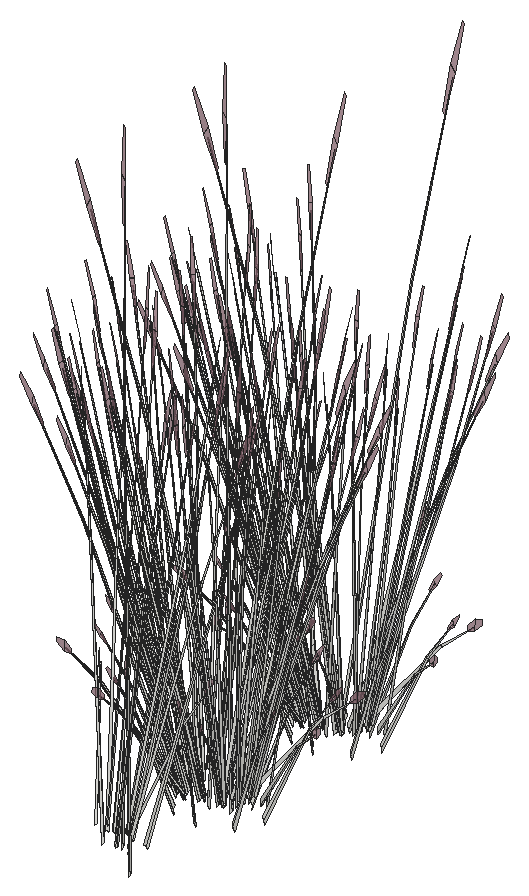
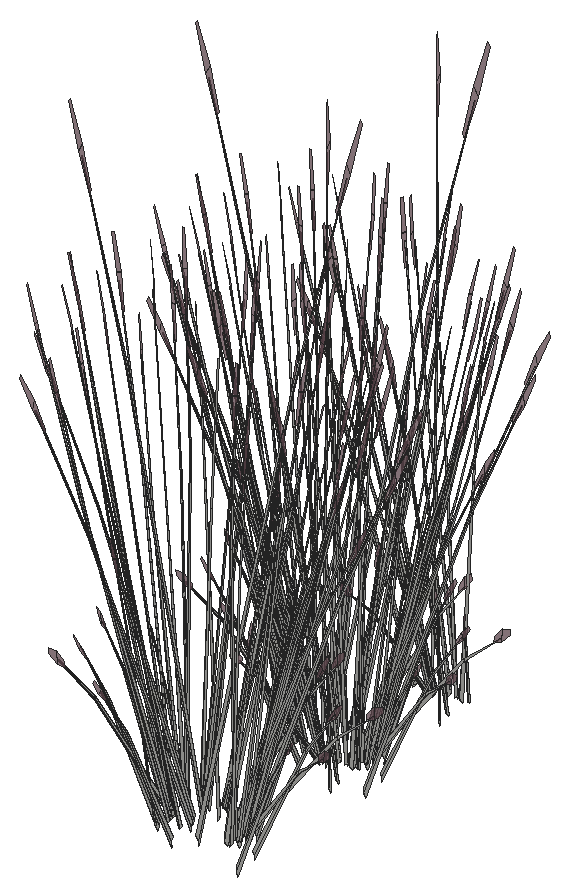
# SketchUp Ruby script. Lengths in inches.
U = 1.inch
M = Sketchup.active_model
def pt(a) = Geom::Point3d.new(a.map { |v| v * U })
def face(e, loops, mat)
  f = e.add_face(loops[0].map { |a| pt(a) })
  loops[1..].each { |l| e.add_face(l.map { |a| pt(a) }).erase! }
  f.material = f.back_material = mat if mat
  f
end
# faces: each face lists its corners as indices into pts; further lists are holes
def faces(e, pts, list, mat = nil) = list.each { |f| face(e, (f[0].is_a?(Array) ? f : [f]).map { |l| l.map { |i| pts[i] } }, mat) }
# xy, xz, yz: faces in a plane at the given z, y or x. An outline is a flat list of corners, or four numbers for a rectangle; further outlines are holes
def ring(l) = l.size == 4 ? [[l[0], l[1]], [l[2], l[1]], [l[2], l[3]], [l[0], l[3]]] : l.each_slice(2).to_a
def flat(e, list, mat, &to3) = list.each { |f| face(e, (f[0].is_a?(Array) ? f : [f]).map { |l| ring(l).map { |u, v| to3.(u, v) } }, mat) }
def xy(e, z, list, mat = nil) = flat(e, list, mat) { |x, y| [x, y, z] }
def xz(e, y, list, mat = nil) = flat(e, list, mat) { |x, z| [x, y, z] }
def yz(e, x, list, mat = nil) = flat(e, list, mat) { |y, z| [x, y, z] }
def lines(e, pts, list) = list.each { |a, b| e.add_line(pt(pts[a]), pt(pts[b])) }
# prism: a flat outline (further loops are holes) pulled along v
def prism(e, loops, v, mat = nil)
  f = face(e, loops, mat); d = Geom::Vector3d.new(v.map { |x| x * U })
  f.pushpull(f.normal.samedirection?(d) ? d.length : -d.length)
end
def box(e, o, s, mat = nil) = prism(e, [[o, [o[0] + s[0], o[1], o[2]], [o[0] + s[0], o[1] + s[1], o[2]], [o[0], o[1] + s[1], o[2]]]], [0, 0, s[2]], mat)
def at(x, y, z, deg = 0) = Geom::Transformation.translation(pt([x, y, z])) * Geom::Transformation.rotation(ORIGIN, Z_AXIS, deg.degrees)
def axes(o, x, y, z) = Geom::Transformation.new([*x, 0, *y, 0, *z, 0, *pt(o).to_a, 1])
def part(name) = M.definitions.add(name)
# library, detail: a bought-in or finely detailed component or shape, given as its bounding box
def library(name, o, s) = part(name).tap { |d| box(d.entities, o, s) }
def detail(e, o, s) = box(e.add_group.entities, o, s)
def put(e, d, t, mat = nil) = e.add_instance(d, t).tap { |i| i.material = mat if mat }
def group(e, t, mat = nil) = e.add_group.tap { |g| g.transformation = t; g.material = mat if mat }.entities
root = M.entities
M.materials.add("LightPink_Translucent").color = [144, 107, 117]
M.materials["LightPink_Translucent"].alpha = 0.75
c1 = part("blade")
p = [[2.15,0.21,22],[0,0.17,0],[0.09,0.45,0],[2.18,0.31,22],[2.29,0.31,22],[0.38,0.45,0],
  [2.48,0.24,33],[2.49,0.24,33],[2.48,0.22,33]]
faces(c1.entities,p,[[0,1,2,3],[4,5,2,3],[6,3,4,7],[8,0,3,6]])
c2 = part("seeds")
p = [[0.3,-0.1,1.38],[-0.01,-0.03,1.59],[-0.01,-0.03,0.03],[0.14,-0.07,-0.07],[0.29,-0.03,3],[0.15,0.01,3.11]]
faces(c2.entities,p,[[0,1,2,3],[1,0,4,5]],"LightPink_Translucent")
c3 = part("blade with seeds")
put(c3.entities,c1,at(0,0,0))
put(c3.entities,c2,axes([2.4,0.25,30.99],[1.5799,-0.05474,1.17369],[-0.12525,1.92788,0.29478],[-0.07173,-0.02425,1.56792]))
put(root,c3,axes([334.74,295.48,50.51],[-0.01379,-0.36791,1.24828],[0.62424,0.09537,0.52853],[-0.14764,0.20132,1.17828]))
put(root,c3,axes([334.79,296.9,52.14],[0.49824,-0.09289,-0.45151],[0.08716,0.35177,-0.34973],[0.13382,0.10081,0.86392]))
put(root,c3,axes([332.16,296.15,51.43],[0.09401,-0.13431,1.51428],[0.3944,0.27795,0.12244],[-0.17792,0.17323,0.64734]))
put(root,c3,axes([332.27,296.91,52],[-0.34164,0.20573,-0.31292],[-0.3234,-0.23491,0.40398],[-0.04921,0.11936,0.77298]))
put(root,c3,axes([331.09,296.85,52.17],[-0.01255,0.07733,1.54581],[0.35618,0.269,-0.24447],[-0.09325,0.12721,0.12397]))
put(root,c3,axes([333.25,297.08,52.45],[0.49409,-0.18193,-0.10745],[0.24281,0.32289,-0.59638],[0.06519,0.13607,0.90619]))
put(root,c3,axes([332.48,297.71,50.44],[-0.01307,-0.23234,1.01491],[0.32652,0.16572,0.74569],[-0.06422,0.11074,0.22354]))
put(root,c3,axes([332.61,296.8125,52.42],[0.36145,0.26255,-0.50118],[-0.38183,0.22994,-0.3882],[-0.055,0.1334,0.95895]))
put(root,c3,axes([333.68,297.07,52.14],[0.49634,0.09796,-0.45151],[-0.17013,0.33585,-0.34973],[0.04551,0.13522,0.86392]))
put(root,c3,axes([333.96,296.37,51.43],[-0.11542,-0.12546,1.51428],[0.53333,-0.10562,0.12244],[0.12054,0.19696,0.64734]))
put(root,c3,axes([333.45,297.27,52],[-0.15222,0.30049,-0.31292],[-0.44409,-0.08764,0.40398],[0.04072,0.12098,0.77298]))
put(root,c3,axes([332.49,296.69,52.72],[-0.01314,0.36145,-0.69681],[-0.55324,-0.02428,0.08409],[-0.05838,0.15313,0.9857]))
put(root,c3,axes([332.69,303.4,51.43],[0.11542,0.12546,1.51428],[-0.53333,0.10562,0.12244],[-0.12054,-0.19696,0.64734]))
put(root,c3,axes([333.02,296.43,51.43],[-0.01236,-0.14998,1.51428],[0.53562,0.09949,0.12244],[-0.03313,0.21373,0.64734]))
put(root,c3,axes([333.57,302.57,52.17],[-0.07723,-0.05479,1.54581],[-0.51538,0.03473,-0.24447],[-0.08225,-0.13104,0.12397]))
put(root,c3,axes([334.11,303.49,52.4],[-0.24099,-0.31773,-0.62776],[0.49607,-0.17707,0.07576],[-0.05635,-0.15352,0.88802]))
put(root,c3,axes([333.5,297,52.4],[0.24099,0.31773,-0.62776],[-0.49607,0.17707,0.07576],[0.05635,0.15352,0.88802]))
put(root,c3,axes([333.14,297.8,52.17],[0.064,0.06292,1.54581],[0.51651,0.02472,-0.24447],[0.05194,0.13877,0.12397]))
put(root,c3,axes([335.12,303.8,52.4],[0.01314,-0.36145,-0.62776],[0.55324,0.02428,0.07576],[0.05838,-0.15313,0.88802]))
put(root,c3,axes([335.89,303.24,52.17],[-0.00487,-0.07777,1.54581],[-0.41166,-0.22476,-0.24447],[0.06364,-0.13625,0.12397]))
put(root,c3,axes([334.16,303.22,52],[0.15222,-0.30049,-0.31292],[0.44409,0.08764,0.40398],[-0.04072,-0.12098,0.77298]))
put(root,c3,axes([334.5,303.62,51.43],[-0.09401,0.13431,1.51428],[-0.3944,-0.27795,0.12244],[0.17792,-0.17323,0.64734]))
put(root,c3,axes([333.93,303.43,52.14],[-0.49634,-0.09796,-0.45151],[0.17013,-0.33585,-0.34973],[-0.04551,-0.13522,0.86392]))
put(root,c3,axes([334.24,302.59,50.44],[0.06477,0.22786,1.01491],[-0.35932,-0.1262,0.74569],[0.03867,-0.11667,0.22354]))
put(root,c3,axes([332.31,297.2,50.97],[0.01109,-0.20172,1.3638],[0.49896,0.10655,0.18846],[-0.04323,0.21498,0.64398]))
put(root,c3,axes([335.01,303.68,52.14],[-0.36145,-0.26255,-0.45151],[0.38183,-0.22994,-0.34973],[0.055,-0.1334,0.86392]))
put(root,c3,axes([334.36,303.41,52.45],[-0.49409,0.18193,-0.10745],[-0.24281,-0.32289,-0.59638],[-0.06519,-0.13607,0.90619]))
put(root,c3,axes([335.38,303.82,52.45],[-0.55492,-0.01936,-0.10745],[0.01517,-0.36657,-0.59638],[0.03855,-0.14118,0.90619]))
put(root,c3,axes([335.35,303.59,52],[0.34164,-0.20573,-0.31292],[0.3234,0.23491,0.40398],[0.04921,-0.11936,0.77298]))
put(root,c3,axes([332.39,302.86,50.44],[0.26338,0.136,1.01491],[-0.38358,0.08175,0.74569],[-0.08207,-0.10452,0.22354]))
put(root,c3,axes([333.03,303.58,52.4],[-0.43054,-0.18887,-0.62776],[0.30598,-0.33097,0.07576],[-0.15599,-0.11277,0.88802]))
put(root,c3,axes([332.88,303.33,52],[-0.07798,-0.31474,-0.31292],[0.44579,-0.08311,0.40398],[-0.11974,-0.09019,0.77298]))
put(root,c3,axes([331.92,303.79,51.43],[0.18755,0.06732,1.51428],[-0.38813,0.28243,0.12244],[-0.24191,-0.12741,0.64734]))
put(root,c3,axes([332.83,303.59,52.14],[-0.49824,0.09289,-0.45151],[-0.08716,-0.35177,-0.34973],[-0.13382,-0.10081,0.86392]))
put(root,c3,axes([335.77,304.43,52.4],[0.26374,-0.30832,-0.62776],[0.46217,0.21911,0.07576],[0.15748,-0.11171,0.88802]))
put(root,c3,axes([335.76,304.29,52.14],[-0.12971,-0.3568,-0.45151],[0.49122,-0.06241,-0.34973],[0.14077,-0.09583,0.86392]))
put(root,c3,axes([331.88,303.17,52.17],[-0.10864,-0.00276,1.54581],[-0.34587,0.27582,-0.24447],[-0.18454,-0.05636,0.12397]))
put(root,c3,axes([335.99,304.54,52.45],[-0.46706,-0.21546,-0.10745],[0.26908,-0.31203,-0.59638],[0.13196,-0.10846,0.90619]))
put(root,c3,axes([334.06,305.72,50.9375],[0.43633,0.15757,1.33654],[-0.42745,0.33945,0.52853],[-0.19146,-0.20119,1.12046]))
put(root,c3,axes([336.36,303.58,50.44],[-0.16818,0.19891,1.01491],[-0.14456,-0.26725,0.74569],[0.1389,-0.06697,0.22354]))
put(root,c3,axes([336.12,304.33,52],[0.43951,-0.05584,-0.31292],[0.11606,0.31924,0.40398],[0.12595,-0.08575,0.77298]))
put(root,c3,axes([331.85,303.89,52],[-0.28729,-0.24465,-0.31292],[0.32804,-0.23159,0.40398],[-0.16667,-0.03524,0.77298]))
put(root,c3,axes([332.15,304.05,52.4],[-0.50473,-0.00941,-0.62776],[0.0339,-0.39618,0.07576],[-0.21383,-0.04181,0.88802]))
put(root,c3,axes([337.39,304.83,52.17],[0.07006,-0.05952,1.54581],[-0.08968,-0.3651,-0.24447],[0.1758,-0.06922,0.12397]))
put(root,c3,axes([331.98,304.13,52.14],[-0.36663,0.25884,-0.45151],[-0.32109,-0.27343,-0.34973],[-0.18628,-0.03938,0.86392]))
put(root,c3,axes([331.16,304.47,50.44],[0.32236,-0.02796,1.01491],[-0.20448,0.24636,0.74569],[-0.1593,-0.03696,0.22354]))
put(root,c3,axes([332.18,303.86,52.45],[-0.02704,0.39739,-0.10745],[-0.51189,-0.01086,-0.59638],[-0.19715,-0.0276,0.90619]))
put(root,c3,axes([336.01,305.38,52.45],[-0.25405,-0.35383,-0.10745],[0.45089,-0.17388,-0.59638],[0.19001,-0.04668,0.90619]))
put(root,c3,axes([335.98,305.08,52.14],[0.13679,-0.35544,-0.45151],[0.46898,0.12183,-0.34973],[0.18882,-0.03259,0.86392]))
put(root,c3,axes([331.52,304.41,51.43],[0.20943,-0.00885,1.51428],[-0.13893,0.38357,0.12244],[-0.29846,-0.02372,0.64734]))
put(root,c3,axes([335.9,305.21,52.4],[0.44368,-0.17257,-0.62776],[0.24726,0.35524,0.07576],[0.21437,-0.04035,0.88802]))
put(root,c3,axes([336.27,305.24,52],[0.41962,0.10901,-0.31292],[-0.12239,0.31802,0.40398],[0.16894,-0.02916,0.77298]))
put(root,c3,axes([331.34,304.74,52],[-0.41962,-0.10901,-0.31292],[0.12239,-0.31802,0.40398],[-0.16894,0.02916,0.77298]))
put(root,c3,axes([335.13,304.85,51.43],[-0.20943,0.00885,1.51428],[0.13893,-0.38357,0.12244],[0.29846,0.02372,0.64734]))
put(root,c3,axes([332.62,304.68,50.95],[0.14352,-0.05653,1.56454],[0.04949,0.39467,0.12244],[-0.31087,0.05237,0.55918]))
put(root,c3,axes([337.16,305.31,50.44],[-0.31197,0.06451,1.01491],[0.14684,-0.26661,0.74569],[0.1655,0.01824,0.22354]))
put(root,c3,axes([331.08,304.95,52.17],[-0.08245,0.05073,1.54581],[0.00701,0.37067,-0.24447],[-0.18899,0.0482,0.12397]))
put(root,c3,axes([331.63,304.9,52.14],[-0.13679,0.35544,-0.45151],[-0.46898,-0.12183,-0.34973],[-0.18882,0.03259,0.86392]))
put(root,c3,axes([331.61,304.59,52.45],[0.25405,0.35383,-0.10745],[-0.45089,0.17388,-0.59638],[-0.19001,0.04668,0.90619]))
put(root,c3,axes([336.62,306.13,51.47],[-0.09664,-0.32847,-0.03085],[0.45676,-0.07551,-0.13989],[0.09538,0.02082,0.4614]))
put(root,c3,axes([335.4375,306.12,52.45],[0.02704,-0.39739,-0.10745],[0.51189,0.01086,-0.59638],[0.19715,0.0276,0.90619]))
put(root,c3,axes([335.88,305.88,52.17],[0.10831,-0.00661,1.54581],[0.29709,-0.30358,-0.24447],[0.19266,0.04007,0.12397]))
put(root,c3,axes([331.61,305.08,51.43],[0.17519,-0.08265,1.51428],[0.14749,0.38193,0.12244],[-0.27504,0.08632,0.64734]))
put(root,c3,axes([335.46,305.93,52.4],[0.50473,0.00941,-0.62776],[-0.0339,0.39618,0.07576],[0.21383,0.04181,0.88802]))
put(root,c3,axes([330.7,306.42,50.44],[0.21042,-0.1771,1.01491],[0.08303,0.28036,0.74569],[-0.15207,0.0502,0.22354]))
put(root,c3,axes([335.77,306.09,52],[0.28729,0.24465,-0.31292],[-0.32804,0.23159,0.40398],[0.16667,0.03524,0.77298]))
put(root,c3,axes([331.49,305.65,52],[-0.43951,0.05584,-0.31292],[-0.11606,-0.31924,0.40398],[-0.12595,0.08575,0.77298]))
put(root,c3,axes([334.73,305.47,51.43],[-0.18755,-0.06732,1.51428],[0.38813,-0.28243,0.12244],[0.24191,0.12741,0.64734]))
put(root,c3,axes([334.77,304.58,51.95],[-0.4363,-0.20303,1.22187],[0.46069,-0.31611,0.5272],[0.14077,0.1905,1.18105]))
put(root,c3,axes([331.625,305.4375,52.45],[0.46706,0.21546,-0.10745],[-0.26908,0.31203,-0.59638],[-0.13196,0.10846,0.90619]))
put(root,c3,axes([335.43,306.23,50.44],[-0.28429,-0.11236,1.01491],[0.36709,-0.11416,0.74569],[0.09901,0.0967,0.22354]))
put(root,c3,axes([334.43,306.55,52.45],[0.30087,-0.33447,-0.10745],[0.43572,0.19269,-0.59638],[0.15146,0.0945,0.90619]))
put(root,c3,axes([332.25,305.34,51.43],[0.12611,-0.12006,1.51428],[0.31843,0.32408,0.12244],[-0.2184,0.14759,0.64734]))
put(root,c3,axes([331.86,305.69,52.14],[0.12971,0.3568,-0.45151],[-0.49122,0.06241,-0.34973],[-0.14077,0.09583,0.86392]))
put(root,c3,axes([334.74,304.97,50.51],[-0.01379,-0.36791,1.24828],[0.62424,0.09537,0.52853],[-0.14764,0.20132,1.17828]))
put(root,c3,axes([334.79,306.39,52.14],[0.49824,-0.09289,-0.45151],[0.08716,0.35177,-0.34973],[0.13382,0.10081,0.86392]))
put(root,c3,axes([332.16,305.64,51.43],[0.09401,-0.13431,1.51428],[0.3944,0.27795,0.12244],[-0.17792,0.17323,0.64734]))
put(root,c3,axes([332.27,306.39,52],[-0.34164,0.20573,-0.31292],[-0.3234,-0.23491,0.40398],[-0.04921,0.11936,0.77298]))
put(root,c3,axes([331.09,306.33,52.17],[-0.01255,0.07733,1.54581],[0.35618,0.269,-0.24447],[-0.09325,0.12721,0.12397]))
put(root,c3,axes([333.25,306.57,52.45],[0.49409,-0.18193,-0.10745],[0.24281,0.32289,-0.59638],[0.06519,0.13607,0.90619]))
put(root,c3,axes([332.48,307.19,50.44],[-0.01307,-0.23234,1.01491],[0.32652,0.16572,0.74569],[-0.06422,0.11074,0.22354]))
put(root,c3,axes([332.61,306.3,52.42],[0.36145,0.26255,-0.50118],[-0.38183,0.22994,-0.3882],[-0.055,0.1334,0.95895]))
put(root,c3,axes([333.68,306.55,52.14],[0.49634,0.09796,-0.45151],[-0.17013,0.33585,-0.34973],[0.04551,0.13522,0.86392]))
put(root,c3,axes([333.96,305.86,51.43],[-0.11542,-0.12546,1.51428],[0.53333,-0.10562,0.12244],[0.12054,0.19696,0.64734]))
put(root,c3,axes([333.45,306.76,52],[-0.15222,0.30049,-0.31292],[-0.44409,-0.08764,0.40398],[0.04072,0.12098,0.77298]))
put(root,c3,axes([332.49,306.18,52.72],[-0.01314,0.36145,-0.69681],[-0.55324,-0.02428,0.08409],[-0.05838,0.15313,0.9857]))
put(root,c3,axes([333.02,305.92,51.43],[-0.01236,-0.14998,1.51428],[0.53562,0.09949,0.12244],[-0.03313,0.21373,0.64734]))
put(root,c3,axes([333.5,306.49,52.4],[0.24099,0.31773,-0.62776],[-0.49607,0.17707,0.07576],[0.05635,0.15352,0.88802]))
put(root,c3,axes([333.14,307.29,52.17],[0.064,0.06292,1.54581],[0.51651,0.02472,-0.24447],[0.05194,0.13877,0.12397]))
put(root,c3,axes([332.31,306.68,50.97],[0.01109,-0.20172,1.3638],[0.49896,0.10655,0.18846],[-0.04323,0.21498,0.64398]))
put(root,c3,axes([332.69,314.39,51.43],[0.11542,0.12546,1.51428],[-0.53333,0.10562,0.12244],[-0.12054,-0.19696,0.64734]))
put(root,c3,axes([333.57,313.56,52.17],[-0.07723,-0.05479,1.54581],[-0.51538,0.03473,-0.24447],[-0.08225,-0.13104,0.12397]))
put(root,c3,axes([334.11,314.48,52.4],[-0.24099,-0.31773,-0.62776],[0.49607,-0.17707,0.07576],[-0.05635,-0.15352,0.88802]))
put(root,c3,axes([335.12,314.79,52.4],[0.01314,-0.36145,-0.62776],[0.55324,0.02428,0.07576],[0.05838,-0.15313,0.88802]))
put(root,c3,axes([335.89,314.23,52.17],[-0.00487,-0.07777,1.54581],[-0.41166,-0.22476,-0.24447],[0.06364,-0.13625,0.12397]))
put(root,c3,axes([334.16,314.21,52],[0.15222,-0.30049,-0.31292],[0.44409,0.08764,0.40398],[-0.04072,-0.12098,0.77298]))
put(root,c3,axes([334.5,314.61,51.43],[-0.09401,0.13431,1.51428],[-0.3944,-0.27795,0.12244],[0.17792,-0.17323,0.64734]))
put(root,c3,axes([333.93,314.42,52.14],[-0.49634,-0.09796,-0.45151],[0.17013,-0.33585,-0.34973],[-0.04551,-0.13522,0.86392]))
put(root,c3,axes([334.24,313.58,50.44],[0.06477,0.22786,1.01491],[-0.35932,-0.1262,0.74569],[0.03867,-0.11667,0.22354]))
put(root,c3,axes([335.01,314.67,52.14],[-0.36145,-0.26255,-0.45151],[0.38183,-0.22994,-0.34973],[0.055,-0.1334,0.86392]))
put(root,c3,axes([334.36,314.4,52.45],[-0.49409,0.18193,-0.10745],[-0.24281,-0.32289,-0.59638],[-0.06519,-0.13607,0.90619]))
put(root,c3,axes([335.38,314.8125,52.45],[-0.55492,-0.01936,-0.10745],[0.01517,-0.36657,-0.59638],[0.03855,-0.14118,0.90619]))
put(root,c3,axes([335.35,314.58,52],[0.34164,-0.20573,-0.31292],[0.3234,0.23491,0.40398],[0.04921,-0.11936,0.77298]))
put(root,c3,axes([332.39,313.85,50.44],[0.26338,0.136,1.01491],[-0.38358,0.08175,0.74569],[-0.08207,-0.10452,0.22354]))
put(root,c3,axes([333.03,314.57,52.4],[-0.43054,-0.18887,-0.62776],[0.30598,-0.33097,0.07576],[-0.15599,-0.11277,0.88802]))
put(root,c3,axes([332.88,314.32,52],[-0.07798,-0.31474,-0.31292],[0.44579,-0.08311,0.40398],[-0.11974,-0.09019,0.77298]))
put(root,c3,axes([331.92,314.78,51.43],[0.18755,0.06732,1.51428],[-0.38813,0.28243,0.12244],[-0.24191,-0.12741,0.64734]))
put(root,c3,axes([332.83,314.58,52.14],[-0.49824,0.09289,-0.45151],[-0.08716,-0.35177,-0.34973],[-0.13382,-0.10081,0.86392]))
put(root,c3,axes([335.77,315.42,52.4],[0.26374,-0.30832,-0.62776],[0.46217,0.21911,0.07576],[0.15748,-0.11171,0.88802]))
put(root,c3,axes([335.76,315.28,52.14],[-0.12971,-0.3568,-0.45151],[0.49122,-0.06241,-0.34973],[0.14077,-0.09583,0.86392]))
put(root,c3,axes([331.88,314.16,52.17],[-0.10864,-0.00276,1.54581],[-0.34587,0.27582,-0.24447],[-0.18454,-0.05636,0.12397]))
put(root,c3,axes([335.99,315.53,52.45],[-0.46706,-0.21546,-0.10745],[0.26908,-0.31203,-0.59638],[0.13196,-0.10846,0.90619]))
put(root,c3,axes([334.06,316.71,50.9375],[0.43633,0.15757,1.33654],[-0.42745,0.33945,0.52853],[-0.19146,-0.20119,1.12046]))
put(root,c3,axes([336.36,314.57,50.44],[-0.16818,0.19891,1.01491],[-0.14456,-0.26725,0.74569],[0.1389,-0.06697,0.22354]))
put(root,c3,axes([336.12,315.32,52],[0.43951,-0.05584,-0.31292],[0.11606,0.31924,0.40398],[0.12595,-0.08575,0.77298]))
put(root,c3,axes([331.85,314.875,52],[-0.28729,-0.24465,-0.31292],[0.32804,-0.23159,0.40398],[-0.16667,-0.03524,0.77298]))
put(root,c3,axes([332.15,315.04,52.4],[-0.50473,-0.00941,-0.62776],[0.0339,-0.39618,0.07576],[-0.21383,-0.04181,0.88802]))
put(root,c3,axes([337.39,315.82,52.17],[0.07006,-0.05952,1.54581],[-0.08968,-0.3651,-0.24447],[0.1758,-0.06922,0.12397]))
put(root,c3,axes([331.98,315.12,52.14],[-0.36663,0.25884,-0.45151],[-0.32109,-0.27343,-0.34973],[-0.18628,-0.03938,0.86392]))
put(root,c3,axes([331.16,315.46,50.44],[0.32236,-0.02796,1.01491],[-0.20448,0.24636,0.74569],[-0.1593,-0.03696,0.22354]))
put(root,c3,axes([332.18,314.85,52.45],[-0.02704,0.39739,-0.10745],[-0.51189,-0.01086,-0.59638],[-0.19715,-0.0276,0.90619]))
put(root,c3,axes([336.01,316.375,52.45],[-0.25405,-0.35383,-0.10745],[0.45089,-0.17388,-0.59638],[0.19001,-0.04668,0.90619]))
put(root,c3,axes([335.98,316.07,52.14],[0.13679,-0.35544,-0.45151],[0.46898,0.12183,-0.34973],[0.18882,-0.03259,0.86392]))
put(root,c3,axes([331.52,315.4,51.43],[0.20943,-0.00885,1.51428],[-0.13893,0.38357,0.12244],[-0.29846,-0.02372,0.64734]))
put(root,c3,axes([335.9,316.2,52.4],[0.44368,-0.17257,-0.62776],[0.24726,0.35524,0.07576],[0.21437,-0.04035,0.88802]))
put(root,c3,axes([336.27,316.23,52],[0.41962,0.10901,-0.31292],[-0.12239,0.31802,0.40398],[0.16894,-0.02916,0.77298]))
put(root,c3,axes([331.34,315.73,52],[-0.41962,-0.10901,-0.31292],[0.12239,-0.31802,0.40398],[-0.16894,0.02916,0.77298]))
put(root,c3,axes([335.13,315.84,51.43],[-0.20943,0.00885,1.51428],[0.13893,-0.38357,0.12244],[0.29846,0.02372,0.64734]))
put(root,c3,axes([332.62,315.67,50.95],[0.14352,-0.05653,1.56454],[0.04949,0.39467,0.12244],[-0.31087,0.05237,0.55918]))
put(root,c3,axes([337.16,316.3,50.44],[-0.31197,0.06451,1.01491],[0.14684,-0.26661,0.74569],[0.1655,0.01824,0.22354]))
put(root,c3,axes([331.08,315.9375,52.17],[-0.08245,0.05073,1.54581],[0.00701,0.37067,-0.24447],[-0.18899,0.0482,0.12397]))
put(root,c3,axes([331.63,315.89,52.14],[-0.13679,0.35544,-0.45151],[-0.46898,-0.12183,-0.34973],[-0.18882,0.03259,0.86392]))
put(root,c3,axes([331.61,315.58,52.45],[0.25405,0.35383,-0.10745],[-0.45089,0.17388,-0.59638],[-0.19001,0.04668,0.90619]))
put(root,c3,axes([336.62,317.12,51.47],[-0.09664,-0.32847,-0.03085],[0.45676,-0.07551,-0.13989],[0.09538,0.02082,0.4614]))
put(root,c3,axes([335.4375,317.11,52.45],[0.02704,-0.39739,-0.10745],[0.51189,0.01086,-0.59638],[0.19715,0.0276,0.90619]))
put(root,c3,axes([335.88,316.87,52.17],[0.10831,-0.00661,1.54581],[0.29709,-0.30358,-0.24447],[0.19266,0.04007,0.12397]))
put(root,c3,axes([331.61,316.07,51.43],[0.17519,-0.08265,1.51428],[0.14749,0.38193,0.12244],[-0.27504,0.08632,0.64734]))
put(root,c3,axes([335.46,316.92,52.4],[0.50473,0.00941,-0.62776],[-0.0339,0.39618,0.07576],[0.21383,0.04181,0.88802]))
put(root,c3,axes([330.7,317.41,50.44],[0.21042,-0.1771,1.01491],[0.08303,0.28036,0.74569],[-0.15207,0.0502,0.22354]))
put(root,c3,axes([335.77,317.08,52],[0.28729,0.24465,-0.31292],[-0.32804,0.23159,0.40398],[0.16667,0.03524,0.77298]))
put(root,c3,axes([331.49,316.64,52],[-0.43951,0.05584,-0.31292],[-0.11606,-0.31924,0.40398],[-0.12595,0.08575,0.77298]))
put(root,c3,axes([334.73,316.45,51.43],[-0.18755,-0.06732,1.51428],[0.38813,-0.28243,0.12244],[0.24191,0.12741,0.64734]))
put(root,c3,axes([334.77,315.57,51.95],[-0.4363,-0.20303,1.22187],[0.46069,-0.31611,0.5272],[0.14077,0.1905,1.18105]))
put(root,c3,axes([331.625,316.42,52.45],[0.46706,0.21546,-0.10745],[-0.26908,0.31203,-0.59638],[-0.13196,0.10846,0.90619]))
put(root,c3,axes([335.43,317.22,50.44],[-0.28429,-0.11236,1.01491],[0.36709,-0.11416,0.74569],[0.09901,0.0967,0.22354]))
put(root,c3,axes([334.43,317.54,52.45],[0.30087,-0.33447,-0.10745],[0.43572,0.19269,-0.59638],[0.15146,0.0945,0.90619]))
put(root,c3,axes([332.25,316.33,51.43],[0.12611,-0.12006,1.51428],[0.31843,0.32408,0.12244],[-0.2184,0.14759,0.64734]))
put(root,c3,axes([331.86,316.68,52.14],[0.12971,0.3568,-0.45151],[-0.49122,0.06241,-0.34973],[-0.14077,0.09583,0.86392]))
